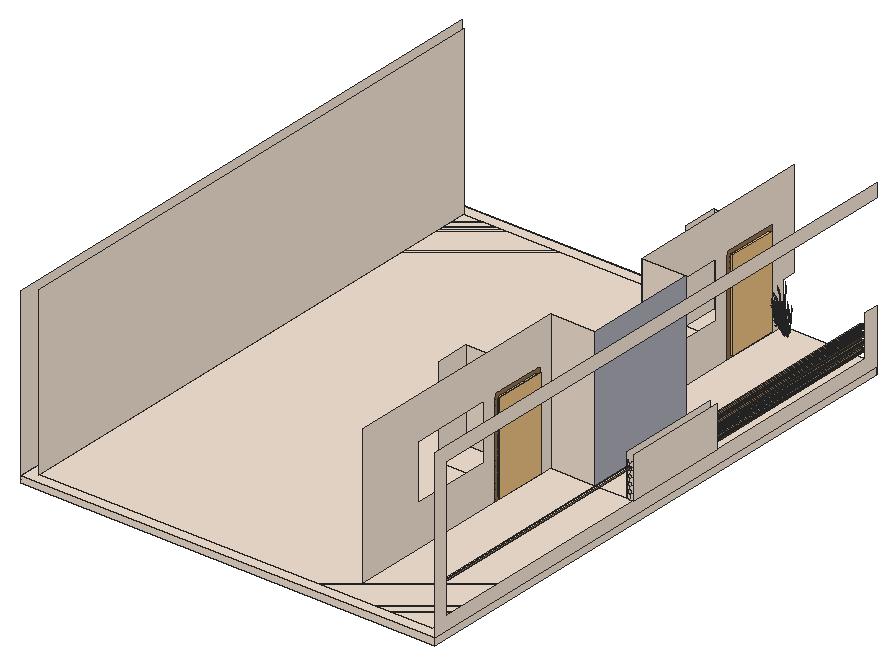
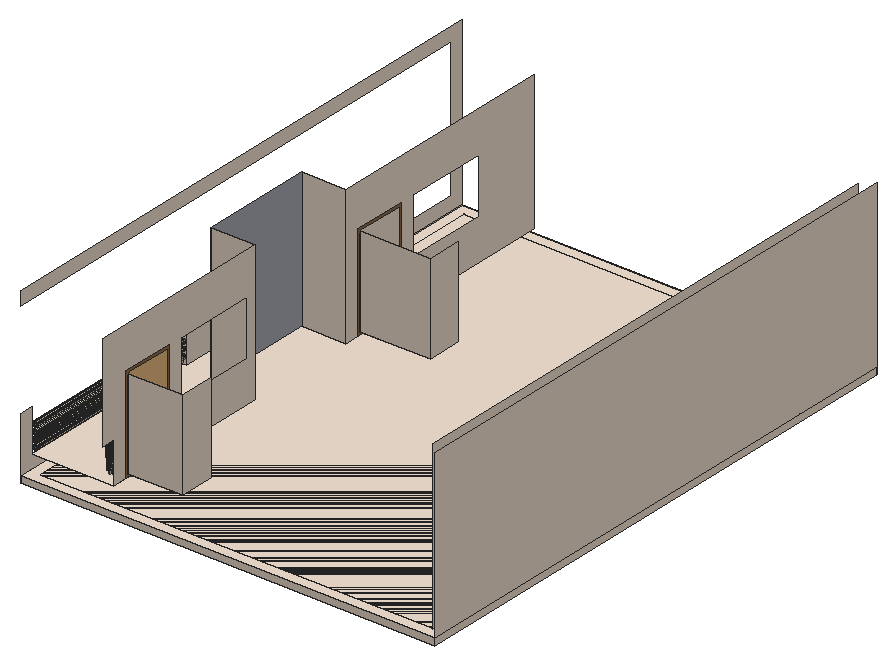
# SketchUp Ruby script. Lengths in inches.
U = 1.inch
M = Sketchup.active_model
def pt(a) = Geom::Point3d.new(a.map { |v| v * U })
def face(e, loops, mat)
  f = e.add_face(loops[0].map { |a| pt(a) })
  loops[1..].each { |l| e.add_face(l.map { |a| pt(a) }).erase! }
  f.material = f.back_material = mat if mat
  f
end
# faces: each face lists its corners as indices into pts; further lists are holes
def faces(e, pts, list, mat = nil) = list.each { |f| face(e, (f[0].is_a?(Array) ? f : [f]).map { |l| l.map { |i| pts[i] } }, mat) }
# xy, xz, yz: faces in a plane at the given z, y or x. An outline is a flat list of corners, or four numbers for a rectangle; further outlines are holes
def ring(l) = l.size == 4 ? [[l[0], l[1]], [l[2], l[1]], [l[2], l[3]], [l[0], l[3]]] : l.each_slice(2).to_a
def flat(e, list, mat, &to3) = list.each { |f| face(e, (f[0].is_a?(Array) ? f : [f]).map { |l| ring(l).map { |u, v| to3.(u, v) } }, mat) }
def xy(e, z, list, mat = nil) = flat(e, list, mat) { |x, y| [x, y, z] }
def xz(e, y, list, mat = nil) = flat(e, list, mat) { |x, z| [x, y, z] }
def yz(e, x, list, mat = nil) = flat(e, list, mat) { |y, z| [x, y, z] }
def lines(e, pts, list) = list.each { |a, b| e.add_line(pt(pts[a]), pt(pts[b])) }
# prism: a flat outline (further loops are holes) pulled along v
def prism(e, loops, v, mat = nil)
  f = face(e, loops, mat); d = Geom::Vector3d.new(v.map { |x| x * U })
  f.pushpull(f.normal.samedirection?(d) ? d.length : -d.length)
end
def box(e, o, s, mat = nil) = prism(e, [[o, [o[0] + s[0], o[1], o[2]], [o[0] + s[0], o[1] + s[1], o[2]], [o[0], o[1] + s[1], o[2]]]], [0, 0, s[2]], mat)
def at(x, y, z, deg = 0) = Geom::Transformation.translation(pt([x, y, z])) * Geom::Transformation.rotation(ORIGIN, Z_AXIS, deg.degrees)
def axes(o, x, y, z) = Geom::Transformation.new([*x, 0, *y, 0, *z, 0, *pt(o).to_a, 1])
def part(name) = M.definitions.add(name)
# library, detail: a bought-in or finely detailed component or shape, given as its bounding box
def library(name, o, s) = part(name).tap { |d| box(d.entities, o, s) }
def detail(e, o, s) = box(e.add_group.entities, o, s)
def put(e, d, t, mat = nil) = e.add_instance(d, t).tap { |i| i.material = mat if mat }
def group(e, t, mat = nil) = e.add_group.tap { |g| g.transformation = t; g.material = mat if mat }.entities
root = M.entities
M.materials.add("C01_Vanilla_Cream").color = [244, 228, 212]
M.materials.add("LightPink_Translucent").color = [144, 107, 117]
M.materials["LightPink_Translucent"].alpha = 0.75
M.materials.add("Marble_20_1K").color = [172, 173, 182]
M.materials.add("Wood_Floor_01_1K").color = [146, 111, 76]
c1 = library("porta+4",[0.2,-5.42,1.33],[46.55,4.72,83.21])
c2 = part("Group\#10")
box(c2.entities,[0,0,0],[360,480,6])
c3 = part("blade")
p = [[2.15,0.21,22],[0,0.17,0],[0.09,0.45,0],[2.18,0.31,22],[2.29,0.31,22],[0.38,0.45,0],
  [2.48,0.24,33],[2.49,0.24,33],[2.48,0.22,33]]
faces(c3.entities,p,[[0,1,2,3],[4,5,2,3],[6,3,4,7],[8,0,3,6]])
c4 = part("seeds")
p = [[0.3,-0.1,1.38],[-0.01,-0.03,1.59],[-0.01,-0.03,0.03],[0.14,-0.07,-0.07],[0.29,-0.03,3],[0.15,0.01,3.11]]
faces(c4.entities,p,[[0,1,2,3],[1,0,4,5]],"LightPink_Translucent")
c5 = part("blade with seeds")
put(c5.entities,c3,at(0,0,0))
put(c5.entities,c4,axes([2.4,0.25,30.99],[1.5799,-0.05474,1.17369],[-0.12525,1.92788,0.29478],[-0.07173,-0.02425,1.56792]))
xy(root,294,[[[0,0,360,480],[9,9,351,471]]],"C01_Vanilla_Cream")
xy(root,300,[[[0,0,360,480],[9,9,351,471]],[9,9,351,471]],"C01_Vanilla_Cream")
xy(root,312,[[326.85,216,354,216,354,306.76,360,306.76,360,468,288,468,288,314.71,326.85,314.71],[354,216,360,306.76]],"C01_Vanilla_Cream")
xy(root,315,[[226.53,171,288,201],[240,423,288,453]],"C01_Vanilla_Cream")
xz(root,201,[[226.53,315,288,393]],"C01_Vanilla_Cream")
xz(root,216,[[288,312,326.85,432],[354,312,357,312,357,316,356.48,316.07,356,316.27,355.59,316.59,355.27,317,355.07,317.48,355,318,354,318],[357,312,360,312,360,318,359,318,358.93,317.48,358.73,317,358.41,316.59,358,316.27,357.52,316.07,357,316],[354,318,355,318,355.07,318.52,355.27,319,355.59,319.41,356,319.73,356.48,319.93,357,320,357,322,356.48,322.07,356,322.27,355.59,322.59,355.27,323,355.07,323.48,355,324,354,324],[359,318,360,318,360,324,359,324,358.93,323.48,358.73,323,358.41,322.59,358,322.27,357.52,322.07,357,322,357,320,357.52,319.93,358,319.73,358.41,319.41,358.73,319,358.93,318.52],
  [354,324,355,324,355.07,324.52,355.27,325,355.59,325.41,356,325.73,356.48,325.93,357,326,357,328,356.48,328.07,356,328.27,355.59,328.59,355.27,329,355.07,329.48,355,330,354,330],[359,324,360,324,360,330,359,330,358.93,329.48,358.73,329,358.41,328.59,358,328.27,357.52,328.07,357,328,357,326,357.52,325.93,358,325.73,358.41,325.41,358.73,325,358.93,324.52],[354,330,355,330,355.07,330.52,355.27,331,355.59,331.41,356,331.73,356.48,331.93,357,332,357,334,356.48,334.07,356,334.27,355.59,334.59,355.27,335,355.07,335.48,355,336,354,336],[359,330,360,330,360,336,359,336,358.93,335.48,358.73,335,358.41,334.59,358,334.27,357.52,334.07,357,334,357,332,357.52,331.93,358,331.73,358.41,331.41,358.73,331,358.93,330.52],[354,336,355,336,355.07,336.52,355.27,337,355.59,337.41,356,337.73,356.48,337.93,357,338,357,340,356.48,340.07,356,340.27,355.59,340.59,355.27,341,355.07,341.48,355,342,354,342],
  [359,336,360,336,360,342,359,342,358.93,341.48,358.73,341,358.41,340.59,358,340.27,357.52,340.07,357,340,357,338,357.52,337.93,358,337.73,358.41,337.41,358.73,337,358.93,336.52]],"C01_Vanilla_Cream")
xz(root,306.76,[[354,312,354,318,355,318,355.07,317.48,355.27,317,355.59,316.59,356,316.27,356.48,316.07,357,316,357,312],[357,312,357,316,357.52,316.07,358,316.27,358.41,316.59,358.73,317,358.93,317.48,359,318,360,318,360,312],[354,318,354,324,355,324,355.07,323.48,355.27,323,355.59,322.59,356,322.27,356.48,322.07,357,322,357,320,356.48,319.93,356,319.73,355.59,319.41,355.27,319,355.07,318.52,355,318],[359,318,358.93,318.52,358.73,319,358.41,319.41,358,319.73,357.52,319.93,357,320,357,322,357.52,322.07,358,322.27,358.41,322.59,358.73,323,358.93,323.48,359,324,360,324,360,318],[354,324,354,330,355,330,355.07,329.48,355.27,329,355.59,328.59,356,328.27,356.48,328.07,357,328,357,326,356.48,325.93,356,325.73,355.59,325.41,355.27,325,355.07,324.52,355,324],
  [359,324,358.93,324.52,358.73,325,358.41,325.41,358,325.73,357.52,325.93,357,326,357,328,357.52,328.07,358,328.27,358.41,328.59,358.73,329,358.93,329.48,359,330,360,330,360,324],[354,330,354,336,355,336,355.07,335.48,355.27,335,355.59,334.59,356,334.27,356.48,334.07,357,334,357,332,356.48,331.93,356,331.73,355.59,331.41,355.27,331,355.07,330.52,355,330],[359,330,358.93,330.52,358.73,331,358.41,331.41,358,331.73,357.52,331.93,357,332,357,334,357.52,334.07,358,334.27,358.41,334.59,358.73,335,358.93,335.48,359,336,360,336,360,330],[354,336,354,342,355,342,355.07,341.48,355.27,341,355.59,340.59,356,340.27,356.48,340.07,357,340,357,338,356.48,337.93,356,337.73,355.59,337.41,355.27,337,355.07,336.52,355,336],[359,336,358.93,336.52,358.73,337,358.41,337.41,358,337.73,357.52,337.93,357,338,357,340,357.52,340.07,358,340.27,358.41,340.59,358.73,341,358.93,341.48,359,342,360,342,360,336]],"C01_Vanilla_Cream")
xz(root,314.71,[[288,312,326.85,432]],"C01_Vanilla_Cream")
xz(root,453,[[240,315,288,393]],"C01_Vanilla_Cream")
yz(root,0,[[0,300,480,444]],"C01_Vanilla_Cream")
yz(root,9,[[9,300,471,444]],"C01_Vanilla_Cream")
yz(root,226.53,[[171,315,201,393]],"C01_Vanilla_Cream")
yz(root,240,[[423,315,453,393]],"C01_Vanilla_Cream")
yz(root,288,[[[12,312,156,312,156,396,204,396,204,312,216,312,216,432,12,432],[72,348,144,396]],[[314.71,312,408,312,408,396,456,396,456,312,468,312,468,348,480,348,480,432,314.71,432],[324,348,396,396]],[159,315,201,393],[411,315,453,393]],"C01_Vanilla_Cream")
yz(root,288,[[[156,312,204,396],[159,315,201,393]],[[408,312,456,396],[411,315,453,393]]],"Wood_Floor_01_1K")
yz(root,326.85,[[216,312,314.71,432]],"Marble_20_1K")
yz(root,354,[[216,312,306.76,348]],"C01_Vanilla_Cream")
yz(root,360,[[0,300,480,300,480,348,468,348,468,312,12,312,12,432,480,432,480,444,0,444],[216,312,306.76,348]],"C01_Vanilla_Cream")
p = [[357,306.76,316],[356.48,306.76,316.07],[356.48,468,316.07],[357,468,316],[357.52,306.76,316.07],[357.52,468,316.07],
  [356,306.76,316.27],[356,468,316.27],[358,306.76,316.27],[358,468,316.27],[355.59,306.76,316.59],[355.59,468,316.59],
  [358.41,306.76,316.59],[358.41,468,316.59],[355.27,306.76,317],[355.27,468,317],[358.73,306.76,317],[358.73,468,317],
  [355.07,306.76,317.48],[355.07,468,317.48],[358.93,306.76,317.48],[358.93,468,317.48],[355,306.76,318],[355,468,318],
  [359,306.76,318],[359,468,318],[355.07,306.76,318.52],[355.07,468,318.52],[358.93,306.76,318.52],[358.93,468,318.52],
  [355.27,306.76,319],[355.27,468,319],[358.73,306.76,319],[358.73,468,319],[355.59,306.76,319.41],[355.59,468,319.41],
  [358.41,306.76,319.41],[358.41,468,319.41],[356,306.76,319.73],[356,468,319.73],[358,306.76,319.73],[358,468,319.73],
  [356.48,306.76,319.93],[356.48,468,319.93],[357.52,306.76,319.93],[357.52,468,319.93],[357,306.76,320],[357,468,320],
  [357,306.76,322],[356.48,306.76,322.07],[356.48,468,322.07],[357,468,322],[357.52,306.76,322.07],[357.52,468,322.07],
  [356,306.76,322.27],[356,468,322.27],[358,306.76,322.27],[358,468,322.27],[355.59,306.76,322.59],[355.59,468,322.59],
  [358.41,306.76,322.59],[358.41,468,322.59],[355.27,306.76,323],[355.27,468,323],[358.73,306.76,323],[358.73,468,323],
  [355.07,306.76,323.48],[355.07,468,323.48],[358.93,306.76,323.48],[358.93,468,323.48],[355,306.76,324],[355,468,324],
  [359,306.76,324],[359,468,324],[355.07,306.76,324.52],[355.07,468,324.52],[358.93,306.76,324.52],[358.93,468,324.52],
  [355.27,306.76,325],[355.27,468,325],[358.73,306.76,325],[358.73,468,325],[355.59,306.76,325.41],[355.59,468,325.41],
  [358.41,306.76,325.41],[358.41,468,325.41],[356,306.76,325.73],[356,468,325.73],[358,306.76,325.73],[358,468,325.73],
  [356.48,306.76,325.93],[356.48,468,325.93],[357.52,306.76,325.93],[357.52,468,325.93],[357,306.76,326],[357,468,326],
  [357,306.76,328],[356.48,306.76,328.07],[356.48,468,328.07],[357,468,328],[357.52,306.76,328.07],[357.52,468,328.07],
  [356,306.76,328.27],[356,468,328.27],[358,306.76,328.27],[358,468,328.27],[355.59,306.76,328.59],[355.59,468,328.59],
  [358.41,306.76,328.59],[358.41,468,328.59],[355.27,306.76,329],[355.27,468,329],[358.73,306.76,329],[358.73,468,329],
  [355.07,306.76,329.48],[355.07,468,329.48],[358.93,306.76,329.48],[358.93,468,329.48],[355,306.76,330],[355,468,330],
  [359,306.76,330],[359,468,330],[355.07,306.76,330.52],[355.07,468,330.52],[358.93,306.76,330.52],[358.93,468,330.52],
  [355.27,306.76,331],[355.27,468,331],[358.73,306.76,331],[358.73,468,331],[355.59,306.76,331.41],[355.59,468,331.41],
  [358.41,306.76,331.41],[358.41,468,331.41],[356,306.76,331.73],[356,468,331.73],[358,306.76,331.73],[358,468,331.73],
  [356.48,306.76,331.93],[356.48,468,331.93],[357.52,306.76,331.93],[357.52,468,331.93],[357,306.76,332],[357,468,332],
  [357,306.76,334],[356.48,306.76,334.07],[356.48,468,334.07],[357,468,334],[357.52,306.76,334.07],[357.52,468,334.07],
  [356,306.76,334.27],[356,468,334.27],[358,306.76,334.27],[358,468,334.27],[355.59,306.76,334.59],[355.59,468,334.59],
  [358.41,306.76,334.59],[358.41,468,334.59],[355.27,306.76,335],[355.27,468,335],[358.73,306.76,335],[358.73,468,335],
  [355.07,306.76,335.48],[355.07,468,335.48],[358.93,306.76,335.48],[358.93,468,335.48],[355,306.76,336],[355,468,336],
  [359,306.76,336],[359,468,336],[355.07,306.76,336.52],[355.07,468,336.52],[358.93,306.76,336.52],[358.93,468,336.52],
  [355.27,306.76,337],[355.27,468,337],[358.73,306.76,337],[358.73,468,337],[358.73,216,337],[358.41,216,337.41],
  [358.41,12,337.41],[358.73,12,337],[355.59,306.76,337.41],[355.59,468,337.41],[358.41,306.76,337.41],[358.41,468,337.41],
  [356,216,337.73],[355.59,216,337.41],[355.59,12,337.41],[356,12,337.73],[358,216,337.73],[358,12,337.73],
  [356,306.76,337.73],[356,468,337.73],[358,306.76,337.73],[358,468,337.73],[356.48,216,337.93],[356.48,12,337.93],
  [357.52,216,337.93],[357.52,12,337.93],[356.48,306.76,337.93],[356.48,468,337.93],[357.52,306.76,337.93],[357.52,468,337.93],
  [357,306.76,338],[357,468,338]]
faces(root,p,[[0,1,2,3],[1,6,7,2],[6,10,11,7],[10,14,15,11],[14,18,19,15],[18,22,23,19],[22,26,27,23],[26,30,31,27],
  [30,34,35,31],[34,38,39,35],[38,42,43,39],[42,46,47,43],[48,49,50,51],[49,54,55,50],[54,58,59,55],[58,62,63,59],
  [62,66,67,63],[66,70,71,67],[70,74,75,71],[74,78,79,75],[78,82,83,79],[82,86,87,83],[86,90,91,87],[90,94,95,91],
  [96,97,98,99],[97,102,103,98],[102,106,107,103],[106,110,111,107],[110,114,115,111],[114,118,119,115],[118,122,123,119],[122,126,127,123],
  [126,130,131,127],[130,134,135,131],[134,138,139,135],[138,142,143,139],[144,145,146,147],[145,150,151,146],[150,154,155,151],[154,158,159,155],
  [158,162,163,159],[162,166,167,163],[166,170,171,167],[170,174,175,171],[174,182,183,175],[186,187,188,189],[182,192,193,183],[196,186,189,197],
  [192,200,201,193],[200,204,205,201]],"C01_Vanilla_Cream")
faces(root,p,[[4,0,3,5],[8,4,5,9],[12,8,9,13],[16,12,13,17],[20,16,17,21],[24,20,21,25],[28,24,25,29],[32,28,29,33],
  [36,32,33,37],[40,36,37,41],[44,40,41,45],[46,44,45,47],[52,48,51,53],[56,52,53,57],[60,56,57,61],[64,60,61,65],
  [68,64,65,69],[72,68,69,73],[76,72,73,77],[80,76,77,81],[84,80,81,85],[88,84,85,89],[92,88,89,93],[94,92,93,95],
  [100,96,99,101],[104,100,101,105],[108,104,105,109],[112,108,109,113],[116,112,113,117],[120,116,117,121],[124,120,121,125],[128,124,125,129],
  [132,128,129,133],[136,132,133,137],[140,136,137,141],[142,140,141,143],[148,144,147,149],[152,148,149,153],[156,152,153,157],[160,156,157,161],
  [164,160,161,165],[168,164,165,169],[172,168,169,173],[176,172,173,177],[178,179,180,181],[184,176,177,185],[179,190,191,180],[194,184,185,195],
  [190,198,199,191],[202,194,195,203],[204,202,203,205]],"Wood_Floor_01_1K")
put(root,c1,axes([289.83,157.29,313.73],[0,0.9504,0],[-0.24166,0,0],[0,0,0.9416]),"C01_Vanilla_Cream")
put(root,c2,at(0,0,294),"C01_Vanilla_Cream")
put(root,c1,axes([291.16,410.82,313.74],[0,0.8978,0],[0.58403,0,0],[0,0,0.94]),"C01_Vanilla_Cream")
put(root,c5,axes([298.18,457.41,314.91],[0.12726,0.15818,1.28532],[-0.58807,0.13317,0.10393],[-0.13291,-0.24832,0.54946]))
put(root,c5,axes([299.16,456.36,315.54],[-0.08515,-0.06907,1.31208],[-0.56828,0.04379,-0.2075],[-0.0907,-0.16522,0.10523]))
put(root,c5,axes([300.47,457.18,313.94],[-0.15825,0.09972,1.07251],[-0.47395,-0.17454,-0.23066],[0.08785,-0.21706,0.45856]))
put(root,c5,axes([299.75,457.52,315.74],[-0.26572,-0.40059,-0.53284],[0.54698,-0.22325,0.0643],[-0.06214,-0.19355,0.75375]))
put(root,c5,axes([298.02,456.99,313.94],[-0.03371,0.16116,1.07251],[-0.49286,0.13491,-0.23066],[-0.11521,-0.20831,0.45856]))
put(root,c5,axes([299.29,456.64,313.12],[-0.09338,0.01775,1.32257],[-0.51641,-0.1998,-0.20205],[0.00867,-0.16666,0.22528]))
put(root,c5,axes([300.86,457.92,315.74],[0.01449,-0.45571,-0.53284],[0.61002,0.03061,0.0643],[0.06438,-0.19306,0.75375]))
put(root,c5,axes([301.71,457.2,315.54],[-0.00537,-0.09805,1.31208],[-0.45391,-0.28338,-0.2075],[0.07018,-0.17178,0.10523]))
put(root,c5,axes([299.8,457.18,315.39],[0.16784,-0.37886,-0.2656],[0.48968,0.1105,0.3429],[-0.0449,-0.15254,0.65611]))
put(root,c5,axes([300.17,457.69,314.91],[-0.10366,0.16934,1.28532],[-0.43488,-0.35044,0.10393],[0.19618,-0.21841,0.54946]))
put(root,c5,axes([301.59,456.85,315.53],[-0.05654,0.03763,1.33037],[-0.55396,-0.12696,-0.12571],[-0.02005,-0.16422,0.23543]))
put(root,c5,axes([299.55,457.44,315.51],[-0.54728,-0.1235,-0.38324],[0.18759,-0.42344,-0.29685],[-0.05018,-0.17048,0.7333]))
put(root,c5,axes([299.89,456.38,314.07],[0.07142,0.28728,0.86145],[-0.3962,-0.15911,0.63294],[0.04263,-0.1471,0.18974]))
put(root,c5,axes([300.73,457.77,315.51],[-0.39855,-0.33102,-0.38324],[0.42102,-0.2899,-0.29685],[0.06064,-0.16819,0.7333]))
put(root,c5,axes([298.57,456.13,315.53],[-0.01039,0.05905,1.33037],[-0.51226,0.21431,-0.12571],[-0.15074,-0.10955,0.23543]))
put(root,c5,axes([298.46,457.18,315.82],[0.62019,-0.12663,0.40322],[0.10763,0.49673,0.33247],[-0.14586,-0.1464,0.83437]))
put(root,c5,axes([299.86,457.27,315.55],[0.54859,0.1288,0.36002],[-0.18759,0.42344,0.29685],[-0.03297,-0.16652,0.74497]))
put(root,c5,axes([300.02,457.42,315.78],[-0.54481,0.22937,-0.0912],[-0.26773,-0.4071,-0.50621],[-0.07188,-0.17155,0.76918]))
put(root,c5,axes([301.15,457.9375,315.78],[-0.61188,-0.02441,-0.0912],[0.01672,-0.46217,-0.50621],[0.0425,-0.178,0.76918]))
put(root,c5,axes([301.11,457.64,315.39],[0.3767,-0.25939,-0.2656],[0.3566,0.29618,0.3429],[0.05426,-0.15048,0.65611]))
put(root,c5,axes([297.85,456.73,314.07],[0.29042,0.17147,0.86145],[-0.42295,0.10307,0.63294],[-0.0905,-0.13178,0.18974]))
put(root,c5,axes([300.01,457.24,315.55],[0.41024,-0.16744,0.04823],[0.2008,0.30532,0.37966],[-0.03962,-0.13459,0.57892]))
put(root,c5,axes([298.55,457.64,315.74],[-0.47473,-0.23813,-0.53284],[0.33738,-0.41728,0.0643],[-0.172,-0.14218,0.75375]))
put(root,c5,axes([298.39,457.32,315.39],[-0.08599,-0.39682,-0.2656],[0.49155,-0.10478,0.3429],[-0.13203,-0.11372,0.65611]))
put(root,c5,axes([298.6,457.29,315.55],[0.25304,-0.31296,0.04823],[0.36033,0.18221,0.37966],[-0.11649,-0.10034,0.57892]))
put(root,c5,axes([297.625,457.25,313.12],[-0.05393,0.0649,1.32257],[-0.545,0.13993,-0.20205],[-0.13166,-0.12729,0.22528]))
put(root,c5,axes([298.52,459.03,313.57],[-0.22864,-0.5052,-0.52377],[0.65862,-0.18195,-0.13747],[-0.02527,-0.17107,1.15612]))
put(root,c5,axes([297.33,457.9,314.91],[0.2068,0.08488,1.28532],[-0.42797,0.35609,0.10393],[-0.26673,-0.16064,0.54946]))
put(root,c5,axes([301.58,457.49,313.12],[-0.08333,-0.03881,1.32257],[-0.21404,-0.4336,-0.20205],[0.14439,-0.11767,0.22528]))
put(root,c5,axes([299.86,457.58,315.79],[-0.16784,0.37886,0.2656],[-0.48968,-0.1105,-0.3429],[-0.0449,-0.15254,0.65611]))
put(root,c5,axes([298.33,457.65,315.51],[-0.54938,0.11711,-0.38324],[-0.0961,-0.44351,-0.29685],[-0.14756,-0.1271,0.7333]))
put(root,c5,axes([301.11,457.74,315.55],[0.39645,0.33614,0.36002],[-0.42102,0.2899,0.29685],[0.07313,-0.15771,0.74497]))
put(root,c5,axes([298.72,457.25,316.07],[-0.37157,0.4723,-0.10215],[-0.5381,-0.2721,-0.56695],[-0.18705,-0.13344,0.86148]))
put(root,c5,axes([301.25,457.78,315.55],[0.45752,0.02296,0.04823],[-0.01254,0.34663,0.37966],[0.04787,-0.13278,0.57892]))
put(root,c5,axes([300.91,458.01,315.79],[-0.3767,0.25939,0.2656],[-0.3566,-0.29618,-0.3429],[0.05426,-0.15048,0.65611]))
put(root,c5,axes([301.58,458.71,315.74],[0.29081,-0.38873,-0.53284],[0.5096,0.27626,0.0643],[0.17364,-0.14084,0.75375]))
put(root,c5,axes([298.43,457.58,313.78],[-0.34808,-0.49367,0],[0.58235,-0.27531,-0.38706],[0.13264,-0.0627,1.22783]))
